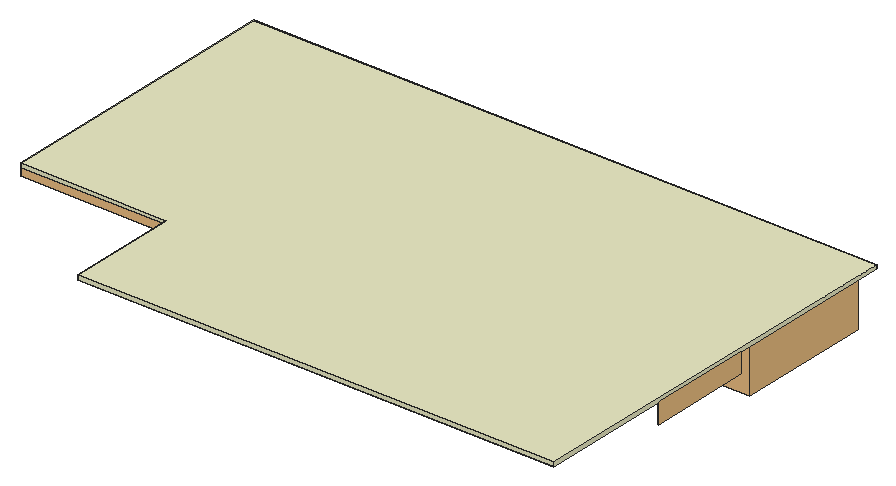
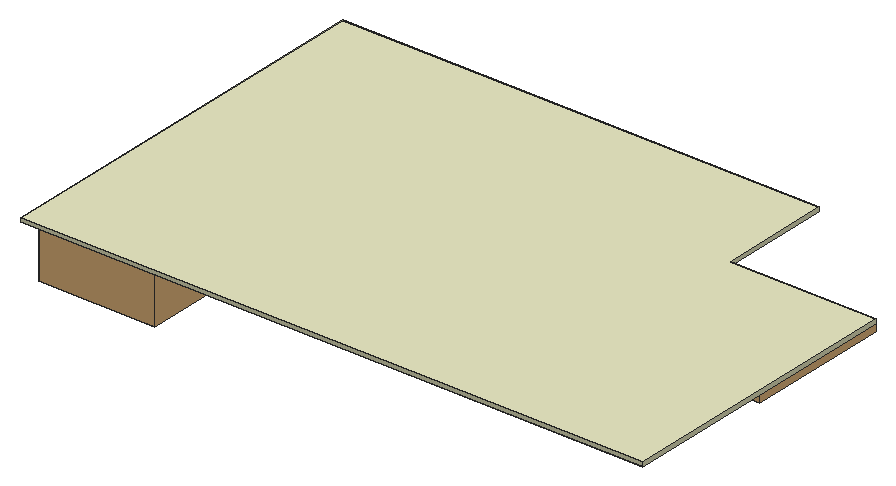
# SketchUp Ruby script. Lengths in inches.
U = 1.inch
M = Sketchup.active_model
def pt(a) = Geom::Point3d.new(a.map { |v| v * U })
def face(e, loops, mat)
  f = e.add_face(loops[0].map { |a| pt(a) })
  loops[1..].each { |l| e.add_face(l.map { |a| pt(a) }).erase! }
  f.material = f.back_material = mat if mat
  f
end
# faces: each face lists its corners as indices into pts; further lists are holes
def faces(e, pts, list, mat = nil) = list.each { |f| face(e, (f[0].is_a?(Array) ? f : [f]).map { |l| l.map { |i| pts[i] } }, mat) }
# xy, xz, yz: faces in a plane at the given z, y or x. An outline is a flat list of corners, or four numbers for a rectangle; further outlines are holes
def ring(l) = l.size == 4 ? [[l[0], l[1]], [l[2], l[1]], [l[2], l[3]], [l[0], l[3]]] : l.each_slice(2).to_a
def flat(e, list, mat, &to3) = list.each { |f| face(e, (f[0].is_a?(Array) ? f : [f]).map { |l| ring(l).map { |u, v| to3.(u, v) } }, mat) }
def xy(e, z, list, mat = nil) = flat(e, list, mat) { |x, y| [x, y, z] }
def xz(e, y, list, mat = nil) = flat(e, list, mat) { |x, z| [x, y, z] }
def yz(e, x, list, mat = nil) = flat(e, list, mat) { |y, z| [x, y, z] }
def lines(e, pts, list) = list.each { |a, b| e.add_line(pt(pts[a]), pt(pts[b])) }
# prism: a flat outline (further loops are holes) pulled along v
def prism(e, loops, v, mat = nil)
  f = face(e, loops, mat); d = Geom::Vector3d.new(v.map { |x| x * U })
  f.pushpull(f.normal.samedirection?(d) ? d.length : -d.length)
end
def box(e, o, s, mat = nil) = prism(e, [[o, [o[0] + s[0], o[1], o[2]], [o[0] + s[0], o[1] + s[1], o[2]], [o[0], o[1] + s[1], o[2]]]], [0, 0, s[2]], mat)
def at(x, y, z, deg = 0) = Geom::Transformation.translation(pt([x, y, z])) * Geom::Transformation.rotation(ORIGIN, Z_AXIS, deg.degrees)
def axes(o, x, y, z) = Geom::Transformation.new([*x, 0, *y, 0, *z, 0, *pt(o).to_a, 1])
def part(name) = M.definitions.add(name)
# library, detail: a bought-in or finely detailed component or shape, given as its bounding box
def library(name, o, s) = part(name).tap { |d| box(d.entities, o, s) }
def detail(e, o, s) = box(e.add_group.entities, o, s)
def put(e, d, t, mat = nil) = e.add_instance(d, t).tap { |i| i.material = mat if mat }
def group(e, t, mat = nil) = e.add_group.tap { |g| g.transformation = t; g.material = mat if mat }.entities
root = M.entities
M.materials.add("1").color = [234, 234, 196]
M.materials.add("[Color_004]").color = [142, 142, 142]
c1 = library("Group\#230",[0,0,-2.65],[191.01,383.01,2.65])
c2 = library("Group\#86",[0,0,0],[154,144,7.49])
c3 = library("Group\#67",[-88.79,0.67,-41.3125],[0.99,6.14,4.87])
c4 = library("Group\#64",[-88.79,21.34,-41.3125],[0.99,6.53,4.87])
c5 = library("Group\#73",[-80.34,-149.03,-93.91],[1.18,2.79,3])
c6 = library("Group\#74",[-80.34,-139.83,-93.89],[1.18,2.84,2.98])
c7 = library("Group\#63",[-80.46,-65.36,-92.6],[1.38,3.58,3.59])
c8 = library("Group\#216",[0,0,0],[114.91,134,52.99])
put(root,c1,axes([1942.23,358,126.79],[0,0,-0.10244],[0,-0.26575,0],[-0.22,0,0]),"1")
put(root,c2,at(1327.72,236.85,119.3),"1")
g1 = group(root,at(1587.08,524.85,126.79),"1")
g2 = group(g1,at(-259.61,0,0))
prism(g2,[[[0,0,0],[615.34,0,0],[615.34,-397.91,0],[144.25,-397.91,0],[144.25,-288,0],[0,-288,0]]],[0,0,4])
g3 = group(root,at(1470.64,328.97,79.75))
detail(g3,[-7.8125,-2.86,-4.27],[0.08,0.65,0.5])
g4 = group(root,at(1470.64,328.97,79.75),"[Color_004]")
prism(g4,[[[-7.73,-1.4375,-4.27],[-7.73,-1.27,-4.27],[-7.73,-1.4,-3.77],[-7.73,-1.61,-3.77],[-7.73,-1.73,-4.11],[-7.73,-1.84,-3.77],[-7.73,-2.04,-3.77],[-7.73,-2.17,-4.27],[-7.73,-2.01,-4.27],[-7.73,-1.92,-3.93],[-7.73,-1.82,-4.27],[-7.73,-1.64,-4.27],[-7.73,-1.53,-3.92]]],[-0.09,0,0],"[Color_004]")
g5 = group(root,at(1470.64,328.97,79.75))
prism(g5,[[[-7.73,-0.82,-4.08],[-7.73,-0.77,-3.96],[-7.73,-1.15,-3.96],[-7.73,-1.23,-4.08]]],[-0.09,0,0],"[Color_004]")
g6 = group(root,at(1470.64,328.97,79.75))
detail(g6,[-7.8125,-1.23,-4.27],[0.08,0.64,0.5])
g7 = group(root,at(1470.64,328.97,79.75))
prism(g7,[[[-7.73,0.02,-3.89],[-7.73,0.02,-3.77],[-7.73,-0.54,-3.77],[-7.73,-0.54,-3.89],[-7.73,-0.36,-3.89],[-7.73,-0.36,-4.27],[-7.73,-0.17,-4.27],[-7.73,-0.17,-3.89]]],[-0.09,0,0],"[Color_004]")
put(root,c3,axes([1470.64,328.97,79.75],[0.088,0,0],[0,0.10336,0],[0,0,0.10336]))
g8 = group(root,at(1470.64,328.97,79.75))
prism(g8,[[[-7.726,1.3,-4.27],[-7.726,1.487,-4.27],[-7.726,1.213,-3.794],[-7.726,1.206,-3.785],[-7.726,1.197,-3.777],[-7.726,1.187,-3.772],[-7.726,1.176,-3.768],[-7.726,1.165,-3.767],[-7.726,1.04,-3.767],[-7.726,1.028,-3.768],[-7.726,1.017,-3.772],[-7.726,1.007,-3.777],[-7.726,0.999,-3.785],[-7.726,0.992,-3.794],[-7.726,0.718,-4.27],[-7.726,0.904,-4.27],[-7.726,0.965,-4.164],[-7.726,1.239,-4.164]],[[-7.726,1.191,-4.08],[-7.726,1.014,-4.08],[-7.726,1.102,-3.927]]],[-0.088,0,0],"[Color_004]")
g9 = group(root,at(1470.64,328.97,79.75))
detail(g9,[-7.8125,1.46,-4.27],[0.08,0.67,0.5])
put(root,c4,axes([1470.64,328.97,79.75],[0.088,0,0],[0,0.10336,0],[0,0,0.10336]))
g10 = group(root,at(1625.625,381.93,79.75),"[Color_004]")
prism(g10,[[[-1.4375,7.73,-4.27],[-1.27,7.73,-4.27],[-1.4,7.73,-3.77],[-1.61,7.73,-3.77],[-1.73,7.73,-4.11],[-1.84,7.73,-3.77],[-2.04,7.73,-3.77],[-2.17,7.73,-4.27],[-2.01,7.73,-4.27],[-1.92,7.73,-3.93],[-1.82,7.73,-4.27],[-1.64,7.73,-4.27],[-1.53,7.73,-3.92]]],[0,0.09,0],"[Color_004]")
put(root,c4,axes([1625.625,381.93,79.75],[0,-0.088,0],[0.10336,0,0],[0,0,0.10336]))
g11 = group(root,at(1625.625,381.93,79.75))
detail(g11,[1.46,7.73,-4.27],[0.67,0.08,0.5])
put(root,c3,axes([1625.625,381.93,79.75],[0,-0.088,0],[0.10336,0,0],[0,0,0.10336]))
g12 = group(root,at(1625.625,381.93,79.75))
detail(g12,[-2.86,7.73,-4.27],[0.65,0.08,0.5])
g13 = group(root,at(1625.625,381.93,79.75))
prism(g13,[[[0.02,7.73,-3.89],[0.02,7.73,-3.77],[-0.54,7.73,-3.77],[-0.54,7.73,-3.89],[-0.36,7.73,-3.89],[-0.36,7.73,-4.27],[-0.17,7.73,-4.27],[-0.17,7.73,-3.89]]],[0,0.09,0],"[Color_004]")
g14 = group(root,at(1625.625,381.93,79.75))
prism(g14,[[[1.3,7.726,-4.27],[1.487,7.726,-4.27],[1.213,7.726,-3.794],[1.206,7.726,-3.785],[1.197,7.726,-3.777],[1.187,7.726,-3.772],[1.176,7.726,-3.768],[1.165,7.726,-3.767],[1.04,7.726,-3.767],[1.028,7.726,-3.768],[1.017,7.726,-3.772],[1.007,7.726,-3.777],[0.999,7.726,-3.785],[0.992,7.726,-3.794],[0.718,7.726,-4.27],[0.904,7.726,-4.27],[0.965,7.726,-4.164],[1.239,7.726,-4.164]],[[1.191,7.726,-4.08],[1.014,7.726,-4.08],[1.102,7.726,-3.927]]],[0,0.088,0],"[Color_004]")
g15 = group(root,at(1625.625,381.93,79.75))
detail(g15,[-1.23,7.73,-4.27],[0.64,0.08,0.5])
g16 = group(root,at(1625.625,381.93,79.75))
prism(g16,[[[-0.82,7.73,-4.08],[-0.77,7.73,-3.96],[-1.15,7.73,-3.96],[-1.23,7.73,-4.08]]],[0,0.09,0],"[Color_004]")
g17 = group(root,at(1533.44,448.8,108.52))
prism(g17,[[[-7.07,-15.5,-9.29],[-7.07,-15.45,-9.6],[-7.07,-15.52,-9.6],[-7.07,-15.57,-9.29]]],[0.1,0,0],"[Color_004]")
g18 = group(root,at(1533.44,448.8,108.52))
detail(g18,[-7.07,-15.51,-9.71],[0.1,0.08,0.08])
put(root,c5,axes([1533.44,448.8,108.52],[0.088,0,0],[0,0.10336,0],[0,0,0.10336]))
g19 = group(root,at(1533.44,448.8,108.52),"[Color_004]")
prism(g19,[[[-7.07,-15.07,-9.4],[-7.07,-14.96,-9.6],[-7.07,-14.92,-9.4],[-7.07,-14.85,-9.4],[-7.07,-14.91,-9.7],[-7.07,-14.98,-9.7],[-7.07,-15.15,-9.4]]],[0.1,0,0],"[Color_004]")
g20 = group(root,at(1533.44,448.8,108.52))
detail(g20,[-7.07,-14.86,-9.37],[0.1,0.08,0.08])
g21 = group(root,at(1533.44,448.8,108.52))
prism(g21,[[[-7.07,-14.79,-9.7],[-7.07,-14.84,-9.4],[-7.07,-14.77,-9.4],[-7.07,-14.72,-9.7]]],[0.1,0,0],"[Color_004]")
g22 = group(root,at(1533.44,448.8,108.52))
detail(g22,[-7.07,-14.73,-9.7],[0.1,0.25,0.41])
put(root,c6,axes([1533.44,448.8,108.52],[0.088,0,0],[0,0.10336,0],[0,0,0.10336]))
put(root,c7,axes([1533.43,448.8,108.52],[0.088,0,0],[0,0.10336,0],[0,0,0.10336]))
g23 = group(root,at(1533.51,448.8,108.52))
detail(g23,[-7.8125,-2.86,-4.27],[0.08,0.65,0.5])
g24 = group(root,at(1533.51,448.8,108.52),"[Color_004]")
prism(g24,[[[-7.73,-1.4375,-4.27],[-7.73,-1.27,-4.27],[-7.73,-1.4,-3.77],[-7.73,-1.61,-3.77],[-7.73,-1.73,-4.11],[-7.73,-1.84,-3.77],[-7.73,-2.04,-3.77],[-7.73,-2.17,-4.27],[-7.73,-2.01,-4.27],[-7.73,-1.92,-3.93],[-7.73,-1.82,-4.27],[-7.73,-1.64,-4.27],[-7.73,-1.53,-3.92]]],[-0.09,0,0],"[Color_004]")
g25 = group(root,at(1533.51,448.8,108.52))
prism(g25,[[[-7.73,-0.82,-4.08],[-7.73,-0.77,-3.96],[-7.73,-1.15,-3.96],[-7.73,-1.23,-4.08]]],[-0.09,0,0],"[Color_004]")
put(root,c8,at(1817.9,380.85,73.8))
